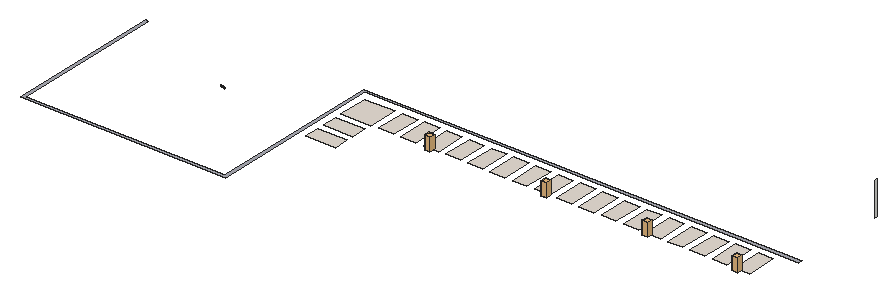
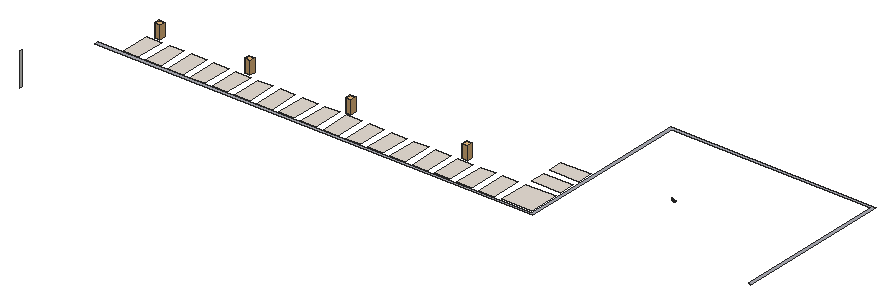
# SketchUp Ruby script. Lengths in inches.
U = 1.inch
M = Sketchup.active_model
def pt(a) = Geom::Point3d.new(a.map { |v| v * U })
def face(e, loops, mat)
  f = e.add_face(loops[0].map { |a| pt(a) })
  loops[1..].each { |l| e.add_face(l.map { |a| pt(a) }).erase! }
  f.material = f.back_material = mat if mat
  f
end
# faces: each face lists its corners as indices into pts; further lists are holes
def faces(e, pts, list, mat = nil) = list.each { |f| face(e, (f[0].is_a?(Array) ? f : [f]).map { |l| l.map { |i| pts[i] } }, mat) }
# xy, xz, yz: faces in a plane at the given z, y or x. An outline is a flat list of corners, or four numbers for a rectangle; further outlines are holes
def ring(l) = l.size == 4 ? [[l[0], l[1]], [l[2], l[1]], [l[2], l[3]], [l[0], l[3]]] : l.each_slice(2).to_a
def flat(e, list, mat, &to3) = list.each { |f| face(e, (f[0].is_a?(Array) ? f : [f]).map { |l| ring(l).map { |u, v| to3.(u, v) } }, mat) }
def xy(e, z, list, mat = nil) = flat(e, list, mat) { |x, y| [x, y, z] }
def xz(e, y, list, mat = nil) = flat(e, list, mat) { |x, z| [x, y, z] }
def yz(e, x, list, mat = nil) = flat(e, list, mat) { |y, z| [x, y, z] }
def lines(e, pts, list) = list.each { |a, b| e.add_line(pt(pts[a]), pt(pts[b])) }
# prism: a flat outline (further loops are holes) pulled along v
def prism(e, loops, v, mat = nil)
  f = face(e, loops, mat); d = Geom::Vector3d.new(v.map { |x| x * U })
  f.pushpull(f.normal.samedirection?(d) ? d.length : -d.length)
end
def box(e, o, s, mat = nil) = prism(e, [[o, [o[0] + s[0], o[1], o[2]], [o[0] + s[0], o[1] + s[1], o[2]], [o[0], o[1] + s[1], o[2]]]], [0, 0, s[2]], mat)
def at(x, y, z, deg = 0) = Geom::Transformation.translation(pt([x, y, z])) * Geom::Transformation.rotation(ORIGIN, Z_AXIS, deg.degrees)
def axes(o, x, y, z) = Geom::Transformation.new([*x, 0, *y, 0, *z, 0, *pt(o).to_a, 1])
def part(name) = M.definitions.add(name)
# library, detail: a bought-in or finely detailed component or shape, given as its bounding box
def library(name, o, s) = part(name).tap { |d| box(d.entities, o, s) }
def detail(e, o, s) = box(e.add_group.entities, o, s)
def put(e, d, t, mat = nil) = e.add_instance(d, t).tap { |i| i.material = mat if mat }
def group(e, t, mat = nil) = e.add_group.tap { |g| g.transformation = t; g.material = mat if mat }.entities
root = M.entities
M.materials.add("Marble_01_1K").color = [230, 221, 211]
M.materials.add("Marble_07_1K").color = [36, 34, 36]
M.materials.add("Marble_20_1K").color = [172, 173, 182]
c1 = library("Group\#54",[0,0,0],[2062.46,2062.46,4833.66])
c2 = part("Landscape+Light")
put(c2.entities,c1,at(-2096.57,-1031.23,-3775.98))
xy(root,2,[[506.43,784.64,554.43,808.64],[506.43,820.64,554.43,844.64],[506.43,856.64,554.43,904.64],[566.43,858.14,590.43,906.14],[602.43,858.14,626.43,906.14],
  [638.43,858.14,662.43,906.14],[674.43,858.14,698.43,906.14],[710.43,858.14,734.43,906.14],[746.43,858.14,770.43,906.14],[782.43,858.14,806.43,906.14],
  [818.43,858.14,842.43,906.14],[854.43,858.14,878.43,906.14],[890.43,858.14,914.43,906.14],[926.43,858.14,950.43,906.14],[962.43,858.14,986.43,906.14],
  [998.43,858.14,1022.43,906.14],[1034.43,858.14,1058.43,906.14],[1070.43,858.14,1094.43,906.14],[1106.43,858.14,1130.43,906.14],[1142.43,858.14,1166.43,906.14]],"Marble_01_1K")
xy(root,6,[[166.21,632.1,498.69,632.1,498.69,913.66,1202.44,913.66,1202.44,918.16,494.19,918.16,494.19,636.6,170.71,636.6,170.71,885.25,166.21,885.25]],"Marble_20_1K")
xz(root,793.34,[[368.27,18,368.28,19]],"Marble_07_1K")
xz(root,795.73,[[362.0625,18,362.15,19]],"Marble_07_1K")
xz(root,795.78,[[361.56,18,361.65,19]],"Marble_07_1K")
yz(root,1204.46,[[1063.52,6,1067.35,60]])
p = [[369.27,792.54,18],[369.23,792.58,18],[369.23,792.58,19],[369.27,792.54,19],[369.32,792.49,18],[369.32,792.49,19],
  [369.18,792.625,18],[369.13,792.67,18],[369.13,792.67,19],[369.18,792.625,19],[369.08,792.71,18],[369.03,792.75,18],
  [369.03,792.75,19],[369.08,792.71,19],[368.99,792.79,18],[368.99,792.79,19],[368.9375,792.83,18],[368.9375,792.83,19],
  [368.89,792.87,18],[368.89,792.87,19],[368.8,792.94,18],[368.75,792.98,18],[368.75,792.98,19],[368.8,792.94,19],
  [368.84,792.91,18],[368.84,792.91,19],[368.7,793.02,18],[368.7,793.02,19],[368.66,793.05,18],[368.66,793.05,19],
  [368.57,793.12,18],[368.53,793.15,18],[368.53,793.15,19],[368.57,793.12,19],[368.5,793.18,18],[368.5,793.18,19],
  [368.61,793.09,18],[368.61,793.09,19],[368.46,793.2,18],[368.43,793.22,18],[368.43,793.22,19],[368.46,793.2,19],
  [368.41,793.24,18],[368.41,793.24,19],[368.38,793.26,18],[368.38,793.26,19],[368.36,793.28,18],[368.35,793.29,18],
  [368.35,793.29,19],[368.36,793.28,19],[368.33,793.3,18],[368.33,793.3,19],[368.32,793.31,18],[368.32,793.31,19],
  [368.3,793.32,18],[368.3,793.32,19],[368.29,793.33,18],[368.29,793.33,19],[368.28,793.34,18],[368.28,793.34,19],
  [368.27,793.34,18],[368.25,793.35,18],[368.25,793.35,19],[368.27,793.34,19],[368.16,793.42,18],[368.125,793.44,18],
  [368.125,793.44,19],[368.16,793.42,19],[368.08,793.47,18],[368.08,793.47,19],[368.24,793.37,18],[368.24,793.37,19],
  [368.22,793.38,18],[368.22,793.38,19],[368.19,793.4,18],[368.19,793.4,19],[367.98,793.55,18],[367.92,793.59,18],
  [367.92,793.59,19],[367.98,793.55,19],[368.03,793.51,18],[368.03,793.51,19],[367.85,793.63,18],[367.78,793.67,18],
  [367.78,793.67,19],[367.85,793.63,19],[367.71,793.72,18],[367.64,793.76,18],[367.64,793.76,19],[367.71,793.72,19],
  [367.57,793.81,18],[367.5,793.85,18],[367.5,793.85,19],[367.57,793.81,19],[367.36,793.9375,18],[367.28,793.98,18],
  [367.28,793.98,19],[367.36,793.9375,19],[367.43,793.9,18],[367.43,793.9,19],[367.21,794.03,18],[367.14,794.07,18],
  [367.14,794.07,19],[367.21,794.03,19],[367.07,794.11,18],[366.99,794.15,18],[366.99,794.15,19],[367.07,794.11,19],
  [366.92,794.19,18],[366.85,794.23,18],[366.85,794.23,19],[366.92,794.19,19],[366.77,794.27,18],[366.77,794.27,19],
  [366.62,794.35,18],[366.55,794.39,18],[366.55,794.39,19],[366.62,794.35,19],[366.7,794.31,18],[366.7,794.31,19],
  [366.47,794.43,18],[366.4,794.46,18],[366.4,794.46,19],[366.47,794.43,19],[366.32,794.5,18],[366.25,794.54,18],
  [366.25,794.54,19],[366.32,794.5,19],[366.17,794.57,18],[366.17,794.57,19],[366.02,794.64,18],[365.94,794.68,18],
  [365.94,794.68,19],[366.02,794.64,19],[366.09,794.61,18],[366.09,794.61,19],[365.79,794.74,18],[365.71,794.78,18],
  [365.71,794.78,19],[365.79,794.74,19],[365.86,794.71,18],[365.86,794.71,19],[365.55,794.84,18],[365.48,794.875,18],
  [365.48,794.875,19],[365.55,794.84,19],[365.63,794.81,18],[365.63,794.81,19],[365.32,794.93,18],[365.24,794.96,18],
  [365.24,794.96,19],[365.32,794.93,19],[365.4,794.9,18],[365.4,794.9,19],[365.08,795.02,18],[365,795.05,18],
  [365,795.05,19],[365.08,795.02,19],[365.16,794.99,18],[365.16,794.99,19],[364.76,795.13,18],[364.68,795.16,18],
  [364.68,795.16,19],[364.76,795.13,19],[364.92,795.08,18],[364.84,795.11,18],[364.84,795.11,19],[364.92,795.08,19],
  [364.52,795.21,18],[364.44,795.24,18],[364.44,795.24,19],[364.52,795.21,19],[364.36,795.26,18],[364.36,795.26,19],
  [364.6,795.1875,18],[364.6,795.1875,19],[364.12,795.33,18],[364.04,795.35,18],[364.04,795.35,19],[364.12,795.33,19],
  [364.2,795.31,18],[364.2,795.31,19],[364.28,795.29,18],[364.28,795.29,19],[363.71,795.4375,18],[363.63,795.46,18],
  [363.63,795.46,19],[363.71,795.4375,19],[363.8,795.42,18],[363.8,795.42,19],[363.88,795.4,18],[363.88,795.4,19],
  [363.96,795.375,18],[363.96,795.375,19],[363.22,795.55,18],[363.14,795.57,18],[363.14,795.57,19],[363.22,795.55,19],
  [363.3,795.53,18],[363.3,795.53,19],[363.39,795.52,18],[363.39,795.52,19],[363.47,795.5,18],[363.47,795.5,19],
  [363.55,795.48,18],[363.55,795.48,19],[362.73,795.64,18],[362.64,795.66,18],[362.64,795.66,19],[362.73,795.64,19],
  [362.81,795.63,18],[362.81,795.63,19],[362.89,795.61,18],[362.89,795.61,19],[362.97,795.6,18],[362.97,795.6,19],
  [363.06,795.58,18],[363.06,795.58,19],[361.98,795.74,18],[361.9,795.75,18],[361.9,795.75,19],[361.98,795.74,19],
  [362.0625,795.73,18],[362.0625,795.73,19],[362.23,795.71,18],[362.15,795.73,18],[362.15,795.73,19],[362.23,795.71,19],
  [362.3125,795.7,18],[362.3125,795.7,19],[362.39,795.69,18],[362.39,795.69,19],[362.48,795.68,18],[362.48,795.68,19],
  [362.56,795.67,18],[362.56,795.67,19],[360.95,795.84,18],[360.83,795.85,18],[360.83,795.85,19],[360.95,795.84,19],
  [361.06,795.83,18],[361.06,795.83,19],[361.17,795.82,18],[361.17,795.82,19],[361.27,795.81,18],[361.27,795.81,19],
  [361.37,795.8,18],[361.37,795.8,19],[361.47,795.79,18],[361.47,795.79,19],[361.56,795.78,18],[361.56,795.78,19],
  [361.73,795.77,18],[361.65,795.78,18],[361.65,795.78,19],[361.73,795.77,19],[361.81,795.76,18],[361.81,795.76,19],
  [360.11,795.95,18],[359.99,795.97,18],[359.99,795.97,19],[360.11,795.95,19],[360.23,795.93,18],[360.23,795.93,19],
  [360.35,795.91,18],[360.35,795.91,19],[360.47,795.89,18],[360.47,795.89,19],[360.59,795.88,18],[360.59,795.88,19],
  [360.71,795.87,18],[360.71,795.87,19],[359.875,795.99,18],[359.76,796.01,18],[359.76,796.01,19],[359.875,795.99,19],
  [368.375,792.51,18],[368.375,792.51,19],[368.33,792.54,18],[368.33,792.54,19],[368.29,792.58,18],[368.29,792.58,19],
  [368.25,792.61,18],[368.25,792.61,19],[368.21,792.64,18],[368.21,792.64,19],[368.17,792.67,18],[368.17,792.67,19],
  [368.13,792.69,18],[368.13,792.69,19],[368.1,792.72,18],[368.1,792.72,19],[368.07,792.74,18],[368.07,792.74,19],
  [368.05,792.76,18],[368.05,792.76,19],[368.03,792.77,18],[368.03,792.77,19],[368.01,792.79,18],[368.01,792.79,19],
  [367.99,792.8,18],[367.99,792.8,19],[367.98,792.8125,18],[367.98,792.8125,19],[367.96,792.82,18],[367.96,792.82,19],
  [367.95,792.83,18],[367.95,792.83,19],[367.9375,792.84,18],[367.9375,792.84,19],[367.93,792.85,18],[367.93,792.85,19],
  [367.92,792.86,18],[367.92,792.86,19],[367.9,792.86,18],[367.9,792.86,19],[367.89,792.875,18],[367.89,792.875,19],
  [367.87,792.89,18],[367.87,792.89,19],[367.84,792.91,18],[367.84,792.91,19],[367.81,792.93,18],[367.81,792.93,19],
  [367.78,792.95,18],[367.78,792.95,19],[367.74,792.98,18],[367.74,792.98,19],[367.69,793.01,18],[367.69,793.01,19],
  [367.64,793.05,18],[367.64,793.05,19],[367.58,793.08,18],[367.58,793.08,19],[367.52,793.125,18],[367.52,793.125,19],
  [367.45,793.17,18],[367.45,793.17,19],[367.39,793.21,18],[367.39,793.21,19],[367.32,793.25,18],[367.32,793.25,19],
  [367.25,793.3,18],[367.25,793.3,19],[367.18,793.34,18],[367.18,793.34,19],[367.11,793.38,18],[367.11,793.38,19],
  [367.05,793.42,18],[367.05,793.42,19],[366.98,793.46,18],[366.98,793.46,19],[366.91,793.5,18],[366.91,793.5,19],
  [366.84,793.54,18],[366.84,793.54,19],[366.77,793.58,18],[366.77,793.58,19],[366.7,793.62,18],[366.7,793.62,19],
  [366.63,793.66,18],[366.63,793.66,19],[366.56,793.7,18],[366.56,793.7,19],[366.49,793.74,18],[366.49,793.74,19],
  [366.42,793.78,18],[366.42,793.78,19],[366.35,793.8125,18],[366.35,793.8125,19],[366.27,793.85,18],[366.27,793.85,19],
  [366.2,793.89,18],[366.2,793.89,19],[366.13,793.92,18],[366.13,793.92,19],[366.06,793.96,18],[366.06,793.96,19],
  [365.99,793.99,18],[365.99,793.99,19],[365.91,794.03,18],[365.91,794.03,19],[365.84,794.06,18],[365.84,794.06,19],
  [365.77,794.09,18],[365.77,794.09,19],[365.69,794.125,18],[365.69,794.125,19],[365.62,794.16,18],[365.62,794.16,19],
  [365.55,794.19,18],[365.55,794.19,19],[365.47,794.22,18],[365.47,794.22,19],[365.4,794.25,18],[365.4,794.25,19],
  [365.33,794.28,18],[365.33,794.28,19],[365.25,794.3125,18],[365.25,794.3125,19],[365.18,794.34,18],[365.18,794.34,19],
  [365.1,794.37,18],[365.1,794.37,19],[365.03,794.4,18],[365.03,794.4,19],[364.95,794.43,18],[364.95,794.43,19],
  [364.875,794.46,18],[364.875,794.46,19],[364.8,794.48,18],[364.8,794.48,19],[364.72,794.51,18],[364.72,794.51,19],
  [364.65,794.54,18],[364.65,794.54,19],[364.57,794.5625,18],[364.57,794.5625,19],[364.5,794.59,18],[364.5,794.59,19],
  [364.42,794.61,18],[364.42,794.61,19],[364.34,794.64,18],[364.34,794.64,19],[364.27,794.66,18],[364.27,794.66,19],
  [364.19,794.68,18],[364.19,794.68,19],[364.11,794.71,18],[364.11,794.71,19],[364.04,794.73,18],[364.04,794.73,19],
  [363.96,794.75,18],[363.96,794.75,19],[363.88,794.77,18],[363.88,794.77,19],[363.8,794.79,18],[363.8,794.79,19],
  [363.73,794.8125,18],[363.73,794.8125,19],[363.65,794.83,18],[363.65,794.83,19],[363.57,794.85,18],[363.57,794.85,19],
  [363.49,794.87,18],[363.49,794.87,19],[363.41,794.89,18],[363.41,794.89,19],[363.34,794.91,18],[363.34,794.91,19],
  [363.26,794.93,18],[363.26,794.93,19],[363.18,794.94,18],[363.18,794.94,19],[363.1,794.96,18],[363.1,794.96,19],
  [363.02,794.97,18],[363.02,794.97,19],[362.94,794.99,18],[362.94,794.99,19],[362.86,795,18],[362.86,795,19],
  [362.79,795.02,18],[362.79,795.02,19],[362.71,795.03,18],[362.71,795.03,19],[362.63,795.05,18],[362.63,795.05,19],
  [362.55,795.06,18],[362.55,795.06,19],[362.47,795.07,18],[362.47,795.07,19],[362.39,795.08,18],[362.39,795.08,19],
  [362.31,795.1,18],[362.31,795.1,19],[362.23,795.11,18],[362.23,795.11,19],[362.15,795.12,18],[362.15,795.12,19],
  [362.07,795.125,18],[362.07,795.125,19],[361.99,795.14,18],[361.99,795.14,19],[361.91,795.14,18],[361.91,795.14,19],
  [361.83,795.15,18],[361.83,795.15,19],[361.75,795.16,18],[361.75,795.16,19],[361.67,795.17,18],[361.67,795.17,19],
  [361.58,795.18,18],[361.58,795.18,19],[361.5,795.18,18],[361.5,795.18,19],[361.41,795.19,18],[361.41,795.19,19],
  [361.3125,795.2,18],[361.3125,795.2,19],[361.21,795.21,18],[361.21,795.21,19],[361.11,795.22,18],[361.11,795.22,19],
  [360.99,795.23,18],[360.99,795.23,19],[360.88,795.24,18],[360.88,795.24,19],[360.76,795.25,18],[360.76,795.25,19],
  [360.64,795.27,18],[360.64,795.27,19],[360.52,795.28,18],[360.52,795.28,19],[360.39,795.3,18],[360.39,795.3,19],
  [360.27,795.3125,18],[360.27,795.3125,19],[360.14,795.33,18],[360.14,795.33,19],[360.02,795.35,18],[360.02,795.35,19],
  [359.89,795.37,18],[359.89,795.37,19],[359.77,795.39,18],[359.77,795.39,19]]
faces(root,p,[[0,1,2,3],[4,0,3,5],[6,7,8,9],[1,6,9,2],[10,11,12,13],[11,14,15,12],[7,10,13,8],[14,16,17,15],
  [16,18,19,17],[20,21,22,23],[18,24,25,19],[24,20,23,25],[21,26,27,22],[26,28,29,27],[30,31,32,33],[31,34,35,32],
  [28,36,37,29],[36,30,33,37],[38,39,40,41],[39,42,43,40],[42,44,45,43],[34,38,41,35],[46,47,48,49],[47,50,51,48],
  [50,52,53,51],[52,54,55,53],[54,56,57,55],[56,58,59,57],[60,61,62,63],[44,46,49,45],[64,65,66,67],[65,68,69,66],
  [61,70,71,62],[70,72,73,71],[72,74,75,73],[74,64,67,75],[76,77,78,79],[68,80,81,69],[80,76,79,81],[82,83,84,85],
  [77,82,85,78],[86,87,88,89],[83,86,89,84],[90,91,92,93],[87,90,93,88],[94,95,96,97],[91,98,99,92],[98,94,97,99],
  [100,101,102,103],[95,100,103,96],[104,105,106,107],[101,104,107,102],[108,109,110,111],[109,112,113,110],[105,108,111,106],[114,115,116,117],
  [118,114,117,119],[112,118,119,113],[120,121,122,123],[115,120,123,116],[124,125,126,127],[125,128,129,126],[121,124,127,122],[130,131,132,133],
  [134,130,133,135],[128,134,135,129],[136,137,138,139],[140,136,139,141],[131,140,141,132],[142,143,144,145],[137,146,147,138],[146,142,145,147],
  [148,149,150,151],[152,148,151,153],[143,152,153,144],[154,155,156,157],[158,154,157,159],[149,158,159,150],[160,161,162,163],[164,165,166,167],
  [165,160,163,166],[155,164,167,156],[168,169,170,171],[169,172,173,170],[174,168,171,175],[161,174,175,162],[176,177,178,179],[180,176,179,181],
  [182,180,181,183],[172,182,183,173],[184,185,186,187],[188,184,187,189],[190,188,189,191],[192,190,191,193],[177,192,193,178],[194,195,196,197],
  [198,194,197,199],[200,198,199,201],[202,200,201,203],[204,202,203,205],[185,204,205,186],[206,207,208,209],[210,206,209,211],[212,210,211,213],
  [214,212,213,215],[216,214,215,217],[195,216,217,196],[218,219,220,221],[222,218,221,223],[224,225,226,227],[228,224,227,229],[230,228,229,231],
  [232,230,231,233],[234,232,233,235],[207,234,235,208],[236,237,238,239],[240,236,239,241],[242,240,241,243],[244,242,243,245],[246,244,245,247],
  [248,246,247,249],[250,248,249,251],[252,253,254,255],[256,252,255,257],[219,256,257,220],[258,259,260,261],[262,258,261,263],[264,262,263,265],
  [266,264,265,267],[268,266,267,269],[270,268,269,271],[237,270,271,238],[272,273,274,275],[259,272,275,260]],"Marble_07_1K")
lines(root,p,[[276,277],[278,279],[280,281],[282,283],[284,285],[286,287],[288,289],[290,291],[292,293],[294,295],[296,297],[298,299],
  [300,301],[302,303],[304,305],[306,307],[308,309],[310,311],[312,313],[314,315],[316,317],[318,319],[320,321],[322,323],
  [324,325],[326,327],[328,329],[330,331],[332,333],[334,335],[336,337],[338,339],[340,341],[342,343],[344,345],[346,347],
  [348,349],[350,351],[352,353],[354,355],[356,357],[358,359],[360,361],[362,363],[364,365],[366,367],[368,369],[370,371],
  [372,373],[374,375],[376,377],[378,379],[380,381],[382,383],[384,385],[386,387],[388,389],[390,391],[392,393],[394,395],
  [396,397],[398,399],[400,401],[402,403],[404,405],[406,407],[408,409],[410,411],[412,413],[414,415],[416,417],[418,419],
  [420,421],[422,423],[424,425],[426,427],[428,429],[430,431],[432,433],[434,435],[436,437],[438,439],[440,441],[442,443],
  [444,445],[446,447],[448,449],[450,451],[452,453],[454,455],[456,457],[458,459],[460,461],[462,463],[464,465],[466,467],
  [468,469],[470,471],[472,473],[474,475],[476,477],[478,479],[480,481],[482,483],[484,485],[486,487],[488,489],[490,491],
  [492,493],[494,495],[496,497],[498,499],[500,501],[502,503],[504,505],[506,507],[508,509],[510,511],[512,513],[514,515],
  [516,517],[518,519],[520,521],[522,523],[524,525]])
put(root,c2,axes([657.53,852.375,20.63],[0.0044,0,0],[0,0.0044,0],[0,0,0.0044]))
put(root,c2,axes([846.49,852.375,20.63],[0.0044,0,0],[0,0.0044,0],[0,0,0.0044]))
put(root,c2,axes([1009.92,852.375,20.63],[0.0044,0,0],[0,0.0044,0],[0,0,0.0044]))
put(root,c2,axes([1155.62,852.375,20.63],[0.0044,0,0],[0,0.0044,0],[0,0,0.0044]))
